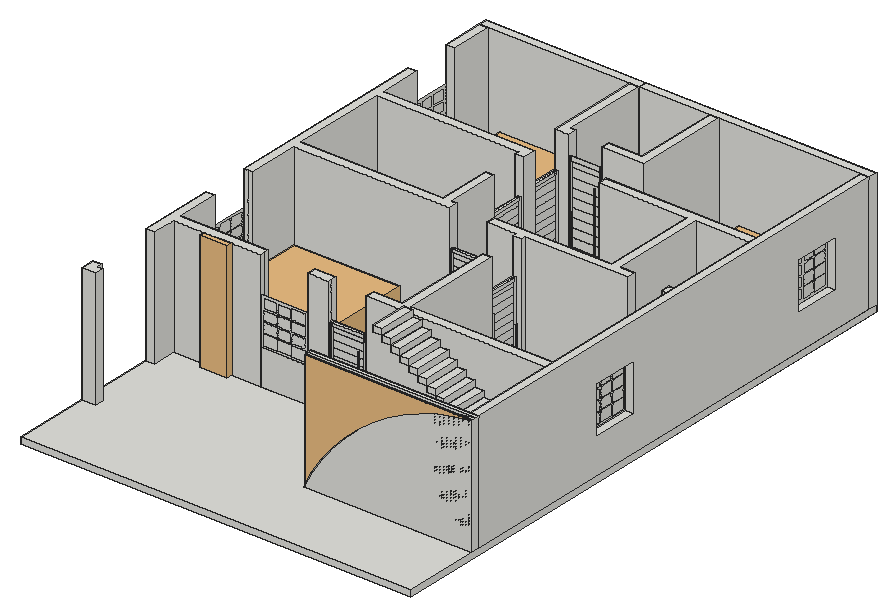
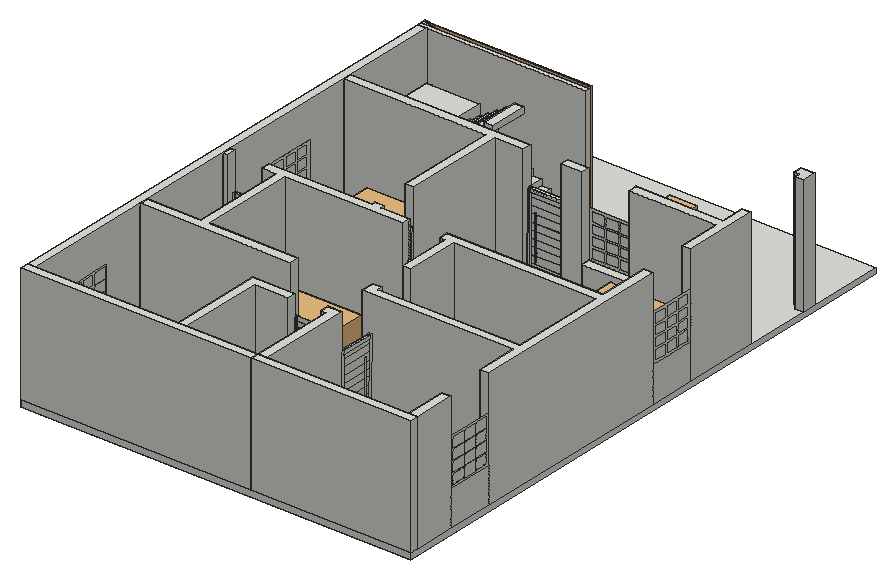
# SketchUp Ruby script. Lengths in inches.
U = 1.inch
M = Sketchup.active_model
def pt(a) = Geom::Point3d.new(a.map { |v| v * U })
def face(e, loops, mat)
  f = e.add_face(loops[0].map { |a| pt(a) })
  loops[1..].each { |l| e.add_face(l.map { |a| pt(a) }).erase! }
  f.material = f.back_material = mat if mat
  f
end
# faces: each face lists its corners as indices into pts; further lists are holes
def faces(e, pts, list, mat = nil) = list.each { |f| face(e, (f[0].is_a?(Array) ? f : [f]).map { |l| l.map { |i| pts[i] } }, mat) }
# xy, xz, yz: faces in a plane at the given z, y or x. An outline is a flat list of corners, or four numbers for a rectangle; further outlines are holes
def ring(l) = l.size == 4 ? [[l[0], l[1]], [l[2], l[1]], [l[2], l[3]], [l[0], l[3]]] : l.each_slice(2).to_a
def flat(e, list, mat, &to3) = list.each { |f| face(e, (f[0].is_a?(Array) ? f : [f]).map { |l| ring(l).map { |u, v| to3.(u, v) } }, mat) }
def xy(e, z, list, mat = nil) = flat(e, list, mat) { |x, y| [x, y, z] }
def xz(e, y, list, mat = nil) = flat(e, list, mat) { |x, z| [x, y, z] }
def yz(e, x, list, mat = nil) = flat(e, list, mat) { |y, z| [x, y, z] }
def lines(e, pts, list) = list.each { |a, b| e.add_line(pt(pts[a]), pt(pts[b])) }
# prism: a flat outline (further loops are holes) pulled along v
def prism(e, loops, v, mat = nil)
  f = face(e, loops, mat); d = Geom::Vector3d.new(v.map { |x| x * U })
  f.pushpull(f.normal.samedirection?(d) ? d.length : -d.length)
end
def box(e, o, s, mat = nil) = prism(e, [[o, [o[0] + s[0], o[1], o[2]], [o[0] + s[0], o[1] + s[1], o[2]], [o[0], o[1] + s[1], o[2]]]], [0, 0, s[2]], mat)
def at(x, y, z, deg = 0) = Geom::Transformation.translation(pt([x, y, z])) * Geom::Transformation.rotation(ORIGIN, Z_AXIS, deg.degrees)
def axes(o, x, y, z) = Geom::Transformation.new([*x, 0, *y, 0, *z, 0, *pt(o).to_a, 1])
def part(name) = M.definitions.add(name)
# library, detail: a bought-in or finely detailed component or shape, given as its bounding box
def library(name, o, s) = part(name).tap { |d| box(d.entities, o, s) }
def detail(e, o, s) = box(e.add_group.entities, o, s)
def put(e, d, t, mat = nil) = e.add_instance(d, t).tap { |i| i.material = mat if mat }
def group(e, t, mat = nil) = e.add_group.tap { |g| g.transformation = t; g.material = mat if mat }.entities
root = M.entities
c1 = part("Agrupar\#4")
xy(c1.entities,0,[[0,0,60.82,4.875]])
c2 = part("Agrupar\#7")
box(c2.entities,[0,0,0.25],[0.65,5.875,0.35])
c3 = part("Agrupar\#15")
prism(c3.entities,[[[0,0.625,0],[0.65,0.625,0],[0.65,0,0],[0,0,0]]],[0,0.02,45.16])
c4 = part("Agrupar\#14")
put(c4.entities,c2,at(0,0.65,6.88))
put(c4.entities,c3,at(0,0,0))
put(c4.entities,c2,at(0,0.65,40.25))
c5 = part("Agrupar\#6")
prism(c5.entities,[[[-0.5,0.62,-4.9375],[0.77,0.62,-4.9375],[0.77,-0.19,-4.9375],[-0.5,-0.19,-4.9375]]],[0,0.03,52.91])
c6 = part("Agrupar\#8")
put(c6.entities,c2,at(0,0.65,6.88))
put(c6.entities,c5,at(0,0,0))
put(c6.entities,c2,at(0,0.65,40.25))
c7 = part("Agrupar\#2")
prism(c7.entities,[[[0,2.67,0.04],[55.46,2.67,0.04],[55.46,0.04,0],[0,0.04,0]]],[0,-0.04,3.23])
c8 = part("Agrupar\#10")
prism(c8.entities,[[[0,3.76,0.04],[4.23,3.76,0.04],[4.23,1.14,0],[0,1.14,0]]],[0,-1.14,83.14])
c9 = part("Agrupar\#1")
prism(c9.entities,[[[0,3.76,0.04],[4.23,3.76,0.04],[4.23,1.14,0],[0,1.14,0]]],[0,-1.14,83.14])
c10 = part("Agrupar\#3")
put(c10.entities,c7,at(4.23,0,79.91))
put(c10.entities,c8,at(59.6875,0,0))
put(c10.entities,c9,at(0,0,0))
c11 = part("Agrupar\#5")
put(c11.entities,c10,axes([0,-1.34,0.11],[1,0,0],[0,3.10443,-0.05961],[0,0.0192,0.99982]))
c12 = part("Agrupar\#9")
put(c12.entities,c4,axes([49.36,10.72,17.77],[1,0,0],[0,-1,0],[0,0,1]))
put(c12.entities,c6,at(49.36,0,17.76))
put(c12.entities,c11,at(0,0.21,0.01))
c13 = part("Agrupar\#11")
box(c13.entities,[0,0,0],[60.82,4.875,7.44])
c14 = part("Agrupar\#12")
put(c14.entities,c13,at(0,0,67.34))
put(c14.entities,c13,at(0,0,44.83))
put(c14.entities,c13,at(0,0,59.9))
put(c14.entities,c13,at(0,0,74.78))
put(c14.entities,c13,at(0,0,52.37))
put(c14.entities,c13,at(0,0,7.53))
put(c14.entities,c13,at(0,0,0))
put(c14.entities,c13,at(0,0,29.95))
put(c14.entities,c13,at(0,0,15.07))
put(c14.entities,c13,at(0,0,22.51))
put(c14.entities,c13,at(0,0,37.39))
c15 = part("Agrupar\#13")
put(c15.entities,c12,at(0,0,0.0625))
put(c15.entities,c14,axes([2.375,5.17,0.15],[1,0,0],[0,0.48232,0.01095],[0,-0.02269,0.99974]))
c16 = part("PORTA PIVOTANDE ENVERNIZADA LUXURY")
p = [[59.6875,-1.28,79.91],[59.6875,-3.1,79.89],[4.23,-1.28,79.91],[4.23,-3.1,79.89]]
lines(c16.entities,p,[[0,1],[2,3]])
put(c16.entities,c1,at(0.13,-2.89,82.23))
put(c16.entities,c15,at(0,-6.8,-0.11))
c17 = library("bed",[0,0,0],[81.24,78.82,29.53])
c18 = library("SOFAS",[-9.33,-51.94,0],[132.18,168.58,37.5625])
c19 = part("Group\#19")
box(c19.entities,[0,0,0],[9,39,6])
c20 = part("Group\#20")
box(c20.entities,[0,0,0],[54,96,10])
c21 = library("Group\#143",[0,0,0],[83.17,58.86,38.65])
c22 = part("Group\#14")
xy(c22.entities,36,[[0,0,9,48]])
yz(c22.entities,0,[[0,0,48,36]])
yz(c22.entities,9,[[0,0,48,36]])
c23 = part("Group\#15")
xy(c23.entities,0,[[0,0,9,48]])
xz(c23.entities,0,[[0,0,9,36]])
xz(c23.entities,48,[[0,0,9,36]])
put(c23.entities,c22,at(0,0,0))
c24 = library("Group\#177",[0,0,0],[170.16,1.375,119.88])
c25 = part("Группа\#53")
xy(c25.entities,0,[[[-6.3,-13.1875,6.3,13.1875],[-4.25,-11.14,4.25,11.14]]])
xy(c25.entities,0.49,[[-3.9375,-10.83,3.9375,10.83]])
xy(c25.entities,0.98,[[[-6.3,-13.1875,6.3,13.1875],[-4.25,-11.14,4.25,11.14]]])
xz(c25.entities,-13.1875,[[-6.3,0,6.3,0.98]])
xz(c25.entities,-10.83,[[-3.9375,0.31,3.9375,0.49],[-3.9375,0.49,3.9375,0.67]])
xz(c25.entities,10.83,[[-3.9375,0.31,3.9375,0.49],[-3.9375,0.49,3.9375,0.67]])
xz(c25.entities,13.1875,[[-6.3,0,6.3,0.98]])
yz(c25.entities,-6.3,[[-13.1875,0,13.1875,0.98]])
yz(c25.entities,-3.9375,[[-10.83,0.31,10.83,0.49],[-10.83,0.49,10.83,0.67]])
yz(c25.entities,3.9375,[[-10.83,0.31,10.83,0.49],[-10.83,0.49,10.83,0.67]])
yz(c25.entities,6.3,[[-13.1875,0,13.1875,0.98]])
p = [[-3.9375,-10.83,0.31],[3.9375,-10.83,0.31],[-4.25,-11.14,0],[-4.25,11.14,0],[4.25,-11.14,0],[4.25,11.14,0],
  [-3.9375,10.83,0.31],[3.9375,10.83,0.31],[-3.9375,-10.83,0.67],[-3.9375,10.83,0.67],[-4.25,-11.14,0.98],[4.25,-11.14,0.98],
  [-4.25,11.14,0.98],[3.9375,-10.83,0.67],[3.9375,10.83,0.67],[4.25,11.14,0.98]]
faces(c25.entities,p,[[0,1,2],[2,3,0],[2,1,4],[5,4,1],[6,0,3],[7,5,1],[3,5,6],[7,6,5],
  [8,9,10],[10,11,8],[10,9,12],[13,8,11],[14,13,11],[14,11,15],[15,12,9],[14,15,9]])
c26 = part("Группа\#45")
xy(c26.entities,0,[[0,0,21.73,35.43]])
xy(c26.entities,29.92,[[0,0,21.73,35.43]])
xz(c26.entities,0,[[0,0,21.73,29.92]])
xz(c26.entities,35.43,[[0,0,21.73,29.92]])
yz(c26.entities,0,[[0,0,35.43,29.92]])
yz(c26.entities,21.73,[[0,0,22.44,29.92],[22.44,0,35.43,3.15],[[22.44,3.15,35.43,29.92],[22.64,3.35,35.24,29.72]]])
put(c26.entities,c25,axes([21.46,28.9375,16.54],[0,1,0],[0,0,1],[1,0,0]))
c27 = library("LIXEIRA INOX DE BANHEIRO",[-4.13,-4.13,0],[8.25,8.24,13.39])
c28 = part("Группа\#59")
xy(c28.entities,0,[[-13.1875,-4.13,13.1875,4.13]])
c29 = part("Panelled cabinet front \#2")
xy(c29.entities,0,[[[-15.55,-6.5,15.55,6.5],[-13.5,-4.45,13.5,4.45]]])
xy(c29.entities,0.98,[[[-15.55,-6.5,15.55,6.5],[-13.5,-4.45,13.5,4.45]]])
xz(c29.entities,-6.5,[[-15.55,0,15.55,0.98]])
xz(c29.entities,-4.13,[[-13.1875,0.31,13.1875,0.67]])
xz(c29.entities,4.13,[[-13.1875,0.31,13.1875,0.67]])
xz(c29.entities,6.5,[[-15.55,0,15.55,0.98]])
yz(c29.entities,-15.55,[[-6.5,0,6.5,0.98]])
yz(c29.entities,-13.1875,[[-4.13,0.31,4.13,0.67]])
yz(c29.entities,13.1875,[[-4.13,0.31,4.13,0.67]])
yz(c29.entities,15.55,[[-6.5,0,6.5,0.98]])
p = [[13.5,-4.45,0],[-13.5,-4.45,0],[13.1875,-4.13,0.31],[-13.1875,-4.13,0.31],[-13.1875,4.13,0.31],[-13.5,4.45,0],
  [13.1875,4.13,0.31],[13.5,4.45,0],[-13.5,4.45,0.98],[-13.5,-4.45,0.98],[-13.1875,-4.13,0.67],[13.5,-4.45,0.98],
  [13.1875,-4.13,0.67],[13.5,4.45,0.98],[-13.1875,4.13,0.67],[13.1875,4.13,0.67]]
faces(c29.entities,p,[[0,1,2],[3,2,1],[4,3,1],[1,5,4],[2,6,0],[0,6,7],[7,4,5],[6,4,7],
  [8,9,10],[11,10,9],[12,10,11],[11,13,12],[10,14,8],[15,12,13],[14,13,8],[14,15,13]])
put(c29.entities,c28,at(0,0,0.49))
c30 = part("Группа\#56")
xy(c30.entities,0,[[[-7.68,-13.1875,7.68,13.1875],[-5.63,-11.14,5.63,11.14]]])
xy(c30.entities,0.49,[[-5.31,-10.83,5.31,10.83]])
xy(c30.entities,0.98,[[[-7.68,-13.1875,7.68,13.1875],[-5.63,-11.14,5.63,11.14]]])
xz(c30.entities,-13.1875,[[-7.68,0,7.68,0.98]])
xz(c30.entities,-10.83,[[-5.31,0.31,5.31,0.49],[-5.31,0.49,5.31,0.67]])
xz(c30.entities,10.83,[[-5.31,0.31,5.31,0.49],[-5.31,0.49,5.31,0.67]])
xz(c30.entities,13.1875,[[-7.68,0,7.68,0.98]])
yz(c30.entities,-7.68,[[-13.1875,0,13.1875,0.98]])
yz(c30.entities,-5.31,[[-10.83,0.31,10.83,0.49],[-10.83,0.49,10.83,0.67]])
yz(c30.entities,5.31,[[-10.83,0.31,10.83,0.49],[-10.83,0.49,10.83,0.67]])
yz(c30.entities,7.68,[[-13.1875,0,13.1875,0.98]])
p = [[-5.31,-10.83,0.31],[5.31,-10.83,0.31],[-5.63,-11.14,0],[-5.63,11.14,0],[5.63,-11.14,0],[5.63,11.14,0],
  [-5.31,10.83,0.31],[5.31,10.83,0.31],[-5.31,-10.83,0.67],[-5.31,10.83,0.67],[-5.63,-11.14,0.98],[5.63,-11.14,0.98],
  [-5.63,11.14,0.98],[5.31,-10.83,0.67],[5.31,10.83,0.67],[5.63,11.14,0.98]]
faces(c30.entities,p,[[0,1,2],[2,3,0],[2,1,4],[5,4,1],[6,0,3],[7,5,1],[3,5,6],[7,6,5],
  [8,9,10],[10,11,8],[10,9,12],[13,8,11],[14,13,11],[14,11,15],[15,12,9],[14,15,9]])
c31 = part("Panelled cabinet front \#1")
xy(c31.entities,0,[[[-7.68,-13.1875,7.68,13.1875],[-5.63,-11.14,5.63,11.14]]])
xy(c31.entities,0.49,[[-5.31,-10.83,5.31,10.83]])
xy(c31.entities,0.98,[[[-7.68,-13.1875,7.68,13.1875],[-5.63,-11.14,5.63,11.14]]])
xz(c31.entities,-13.1875,[[-7.68,0,7.68,0.98]])
xz(c31.entities,-10.83,[[-5.31,0.31,5.31,0.49],[-5.31,0.49,5.31,0.67]])
xz(c31.entities,10.83,[[-5.31,0.31,5.31,0.49],[-5.31,0.49,5.31,0.67]])
xz(c31.entities,13.1875,[[-7.68,0,7.68,0.98]])
yz(c31.entities,-7.68,[[-13.1875,0,13.1875,0.98]])
yz(c31.entities,-5.31,[[-10.83,0.31,10.83,0.49],[-10.83,0.49,10.83,0.67]])
yz(c31.entities,5.31,[[-10.83,0.31,10.83,0.49],[-10.83,0.49,10.83,0.67]])
yz(c31.entities,7.68,[[-13.1875,0,13.1875,0.98]])
p = [[-5.31,-10.83,0.31],[5.31,-10.83,0.31],[-5.63,-11.14,0],[-5.63,11.14,0],[5.63,-11.14,0],[5.63,11.14,0],
  [-5.31,10.83,0.31],[5.31,10.83,0.31],[-5.63,-11.14,0.98],[5.63,-11.14,0.98],[-5.31,-10.83,0.67],[-5.31,10.83,0.67],
  [-5.63,11.14,0.98],[5.31,-10.83,0.67],[5.31,10.83,0.67],[5.63,11.14,0.98]]
faces(c31.entities,p,[[0,1,2],[2,3,0],[2,1,4],[5,4,1],[6,0,3],[7,5,1],[3,5,6],[7,6,5],
  [8,9,10],[10,11,8],[8,11,12],[13,10,9],[14,13,9],[14,9,15],[15,12,11],[14,15,11]])
c32 = part("Группа\#52")
xy(c32.entities,0,[[[-5.71,-13.1875,5.71,13.1875],[-3.66,-11.14,3.66,11.14]]])
xy(c32.entities,0.49,[[-3.35,-10.83,3.35,10.83]])
xy(c32.entities,0.98,[[[-5.71,-13.1875,5.71,13.1875],[-3.66,-11.14,3.66,11.14]]])
xz(c32.entities,-13.1875,[[-5.71,0,5.71,0.98]])
xz(c32.entities,-10.83,[[-3.35,0.31,3.35,0.49],[-3.35,0.49,3.35,0.67]])
xz(c32.entities,10.83,[[-3.35,0.31,3.35,0.49],[-3.35,0.49,3.35,0.67]])
xz(c32.entities,13.1875,[[-5.71,0,5.71,0.98]])
yz(c32.entities,-5.71,[[-13.1875,0,13.1875,0.98]])
yz(c32.entities,-3.35,[[-10.83,0.31,10.83,0.49],[-10.83,0.49,10.83,0.67]])
yz(c32.entities,3.35,[[-10.83,0.31,10.83,0.49],[-10.83,0.49,10.83,0.67]])
yz(c32.entities,5.71,[[-13.1875,0,13.1875,0.98]])
p = [[3.66,-11.14,0],[-3.66,-11.14,0],[-3.35,-10.83,0.31],[-3.66,11.14,0],[3.35,-10.83,0.31],[3.66,11.14,0],
  [-3.35,10.83,0.31],[3.35,10.83,0.31],[-3.66,11.14,0.98],[-3.66,-11.14,0.98],[-3.35,10.83,0.67],[-3.35,-10.83,0.67],
  [3.35,-10.83,0.67],[3.66,-11.14,0.98],[3.35,10.83,0.67],[3.66,11.14,0.98]]
faces(c32.entities,p,[[0,1,2],[3,2,1],[4,0,2],[5,0,4],[6,2,3],[7,5,4],[3,5,6],[7,6,5],
  [8,9,10],[11,10,9],[12,11,9],[12,9,13],[14,12,13],[13,15,14],[10,14,8],[8,14,15]])
c33 = part("Группа\#54")
xy(c33.entities,0,[[[-6.4,-13.1875,6.4,13.1875],[-4.35,-11.14,4.35,11.14]]])
xy(c33.entities,0.49,[[-4.04,-10.83,4.04,10.83]])
xy(c33.entities,0.98,[[[-6.4,-13.1875,6.4,13.1875],[-4.35,-11.14,4.35,11.14]]])
xz(c33.entities,-13.1875,[[-6.4,0,6.4,0.98]])
xz(c33.entities,-10.83,[[-4.04,0.31,4.04,0.49],[-4.04,0.49,4.04,0.67]])
xz(c33.entities,10.83,[[-4.04,0.31,4.04,0.49],[-4.04,0.49,4.04,0.67]])
xz(c33.entities,13.1875,[[-6.4,0,6.4,0.98]])
yz(c33.entities,-6.4,[[-13.1875,0,13.1875,0.98]])
yz(c33.entities,-4.04,[[-10.83,0.31,10.83,0.49],[-10.83,0.49,10.83,0.67]])
yz(c33.entities,4.04,[[-10.83,0.31,10.83,0.49],[-10.83,0.49,10.83,0.67]])
yz(c33.entities,6.4,[[-13.1875,0,13.1875,0.98]])
p = [[4.35,-11.14,0],[-4.35,-11.14,0],[-4.04,-10.83,0.31],[-4.04,10.83,0.31],[-4.35,11.14,0],[4.04,-10.83,0.31],
  [4.35,11.14,0],[4.04,10.83,0.31],[-4.35,11.14,0.98],[-4.35,-11.14,0.98],[-4.04,-10.83,0.67],[4.35,-11.14,0.98],
  [4.04,-10.83,0.67],[4.35,11.14,0.98],[-4.04,10.83,0.67],[4.04,10.83,0.67]]
faces(c33.entities,p,[[0,1,2],[3,2,1],[1,4,3],[5,0,2],[6,0,7],[5,7,0],[6,3,4],[7,3,6],
  [8,9,10],[11,10,9],[12,10,11],[13,12,11],[10,14,8],[15,12,13],[13,8,15],[14,15,8]])
c34 = library("Inodoro ROCA Meridian-N compact",[-14.68,0,0],[14.68,23.62,31.16])
c35 = library("Grupo\#25",[0.45,21.05,9.1],[4.32,4.21,6.93])
c36 = library("00230906_3D_ducha_hig.dwg\#1",[121.96,-107.5,-116.36],[35.26,104.03,274.49])
c37 = library("Gruppe\#2",[0,-1.9,0],[31.7,22.18,26.07])
c38 = part("Группа\#84")
prism(c38.entities,[[[-19.46,0,0],[-144,0,0],[-144,47.24,0],[-120.375,47.24,0],[-120.375,23.62,0],[-19.46,23.62,0]],[[-81.02,2.55,0],[-81.02,20.78,0],[-106.12,20.78,0],[-106.12,2.55,0]]],[0,0,1.57])
c39 = library("Group\#136",[0,0,0],[7.4375,14.82,1.97])
c40 = library("Group\#138",[0,0,0],[10.4375,12.4,1.97])
c41 = library("Group\#135",[0,0,0],[5.12,5.12,1.0625])
c42 = library("Group\#137",[0,0,0],[7.4375,14.82,1.97])
c43 = part("window_2")
xz(c43.entities,0,[[[-16,0,16,41],[-14,30.25,-5.25,39],[5.25,30.25,14,39],[5.25,2,14,10.75],[-14,2,-5.25,10.75],[-4.25,30.25,4.25,39],[-4.25,2,4.25,10.75],[5.25,21,14,29.25],[5.25,11.75,14,20],[-14,21,-5.25,29.25],[-14,11.75,-5.25,20],[-4.25,21,4.25,29.25],[-4.25,11.75,4.25,20]],[-14,2,-5.25,10.75],[-4.25,2,4.25,10.75],[5.25,2,14,10.75],[-14,11.75,-5.25,20],
  [-4.25,11.75,4.25,20],[5.25,11.75,14,20],[-14,21,-5.25,29.25],[-4.25,21,4.25,29.25],[5.25,21,14,29.25],
  [-14,30.25,-5.25,39],[-4.25,30.25,4.25,39],[5.25,30.25,14,39]])
c44 = library("Gruppe\#1",[0,0,0],[10.625,1.33,3.5625])
c45 = part("Component\#35")
detail(c45.entities,[0,0,0],[0.1,0.79,0.125])
c46 = library("Component\#38",[0,0,0],[0.16,0.16,0.04])
prism(root,[[[52.638,387.274,41.253],[52.658,387.274,41.25],[52.679,387.274,41.253],[52.698,387.274,41.261],[52.714,387.274,41.273],[52.726,387.274,41.289],[52.734,387.274,41.308],[52.737,387.274,41.329],[52.734,387.274,41.349],[52.726,387.274,41.368],[52.714,387.274,41.384],[52.698,387.274,41.397],[52.679,387.274,41.405],[52.658,387.274,41.407],[52.638,387.274,41.405],[52.619,387.274,41.397],[52.602,387.274,41.384],[52.59,387.274,41.368],[52.582,387.274,41.349],[52.579,387.274,41.329],[52.582,387.274,41.308],[52.59,387.274,41.289],[52.602,387.274,41.273],[52.619,387.274,41.261]]],[0,-0.002,0])
prism(root,[[[56.178,387.274,41.263],[56.199,387.274,41.26],[56.219,387.274,41.263],[56.238,387.274,41.27],[56.254,387.274,41.283],[56.267,387.274,41.299],[56.275,387.274,41.318],[56.278,387.274,41.339],[56.275,387.274,41.359],[56.267,387.274,41.378],[56.254,387.274,41.394],[56.238,387.274,41.407],[56.219,387.274,41.415],[56.199,387.274,41.417],[56.178,387.274,41.415],[56.159,387.274,41.407],[56.143,387.274,41.394],[56.131,387.274,41.378],[56.123,387.274,41.359],[56.12,387.274,41.339],[56.123,387.274,41.318],[56.131,387.274,41.299],[56.143,387.274,41.283],[56.159,387.274,41.27]]],[0,-0.002,0])
prism(root,[[[59.719,387.274,41.272],[59.739,387.274,41.27],[59.76,387.274,41.272],[59.779,387.274,41.28],[59.795,387.274,41.293],[59.808,387.274,41.309],[59.816,387.274,41.328],[59.818,387.274,41.348],[59.816,387.274,41.369],[59.808,387.274,41.388],[59.795,387.274,41.404],[59.779,387.274,41.417],[59.76,387.274,41.424],[59.739,387.274,41.427],[59.719,387.274,41.424],[59.7,387.274,41.417],[59.684,387.274,41.404],[59.671,387.274,41.388],[59.663,387.274,41.369],[59.661,387.274,41.348],[59.663,387.274,41.328],[59.671,387.274,41.309],[59.684,387.274,41.293],[59.7,387.274,41.28]]],[0,-0.002,0])
xy(root,0,[[257.25,120,428.25,129]])
xy(root,26.378,[[109.514,386.793,109.675,386.814,109.825,386.876,109.954,386.975,110.052,387.104,110.115,387.254,110.136,387.415,110.115,387.576,110.052,387.726,109.954,387.855,109.825,387.954,109.675,388.016,109.514,388.037,109.353,388.016,109.203,387.954,109.074,387.855,108.975,387.726,108.913,387.576,108.892,387.415,108.913,387.254,108.975,387.104,109.074,386.975,109.203,386.876,109.353,386.814]])
xy(root,26.772,[[[109.514,386.628,109.718,386.654,109.908,386.733,110.071,386.858,110.196,387.021,110.274,387.211,110.301,387.415,110.274,387.619,110.196,387.809,110.071,387.972,109.908,388.097,109.718,388.176,109.514,388.202,109.31,388.176,109.12,388.097,108.957,387.972,108.832,387.809,108.753,387.619,108.726,387.415,108.753,387.211,108.832,387.021,108.957,386.858,109.12,386.733,109.31,386.654],[109.514,386.793,109.353,386.814,109.203,386.876,109.074,386.975,108.975,387.104,108.913,387.254,108.892,387.415,108.913,387.576,108.975,387.726,109.074,387.855,109.203,387.954,109.353,388.016,109.514,388.037,109.675,388.016,109.825,387.954,109.954,387.855,110.052,387.726,110.115,387.576,110.136,387.415,110.115,387.254,110.052,387.104,109.954,386.975,109.825,386.876,109.675,386.814]]])
xy(root,120,[[257.25,124.5625,428.25,129]])
xz(root,120,[[257.25,0,428.25,0,428.25,120,410.262,117.372,392.561,113.229,375.275,107.599,358.529,100.525,342.443,92.056,327.133,82.255,312.709,71.19,299.274,58.942,286.927,45.6,275.755,31.259,265.839,16.022]])
xz(root,124.5625,[[257.25,0,265.839,16.022,275.755,31.259,286.927,45.6,299.274,58.942,312.709,71.19,327.133,82.255,342.443,92.056,358.529,100.525,375.275,107.599,392.561,113.229,410.262,117.372,428.25,120,257.25,120]])
xz(root,129,[[257.25,0,428.25,120]])
xz(root,422.433,[[41.25,0,62.982,3.15],[41.25,3.15,62.982,29.921]])
xz(root,534,[[32.25,0,41.25,36]])
xz(root,582,[[32.25,0,41.25,36]])
yz(root,62.982,[[[422.433,3.15,434.244,29.921],[422.63,3.346,434.047,29.724]]])
yz(root,143.548,[[405.828,32.839,405.823,32.841,405.97,33.413,405.975,33.411],[405.823,32.841,404.574,33.161,404.721,33.733,405.97,33.413]])
yz(root,143.862,[[405.826,32.84,405.973,33.412,405.97,33.413,405.823,32.841],[405.823,32.841,405.97,33.413,404.717,33.734,404.57,33.162]])
yz(root,257.25,[[124.5625,0,129,120]])
yz(root,428.25,[[120,0,129,120]])
p = [[257.25,120,0],[265.839,120,16.022],[265.839,124.5625,16.022],[257.25,124.5625,0],[275.755,120,31.259],[275.755,124.5625,31.259],
  [109.203,386.876,26.772],[109.353,386.814,26.772],[109.353,386.814,26.378],[109.203,386.876,26.378],[109.514,386.793,26.772],[109.514,386.793,26.378],
  [109.675,386.814,26.772],[109.675,386.814,26.378],[109.825,386.876,26.772],[109.825,386.876,26.378],[109.074,386.975,26.772],[109.074,386.975,26.378],
  [109.954,386.975,26.772],[109.954,386.975,26.378],[108.975,387.104,26.772],[108.975,387.104,26.378],[110.052,387.104,26.772],[110.052,387.104,26.378],
  [108.913,387.254,26.772],[108.913,387.254,26.378],[110.115,387.254,26.772],[110.115,387.254,26.378],[108.892,387.415,26.772],[108.892,387.415,26.378],
  [110.136,387.415,26.772],[110.136,387.415,26.378],[108.913,387.576,26.772],[108.913,387.576,26.378],[110.115,387.576,26.772],[110.115,387.576,26.378],
  [108.975,387.726,26.772],[108.975,387.726,26.378],[110.052,387.726,26.772],[110.052,387.726,26.378],[109.074,387.855,26.772],[109.074,387.855,26.378],
  [109.954,387.855,26.772],[109.954,387.855,26.378],[109.203,387.954,26.772],[109.203,387.954,26.378],[109.825,387.954,26.772],[109.825,387.954,26.378],
  [109.353,388.016,26.772],[109.353,388.016,26.378],[109.514,388.037,26.772],[109.514,388.037,26.378],[109.675,388.016,26.772],[109.675,388.016,26.378],
  [286.927,120,45.6],[286.927,124.5625,45.6],[143.114,404.798,32.697],[143.054,404.957,32.657],[143.037,405.125,32.613],[143.066,405.292,32.571],
  [143.139,405.446,32.531],[143.25,405.577,32.498],[143.393,405.675,32.472],[143.557,405.734,32.457],[143.73,405.75,32.453],[143.903,405.721,32.46],
  [144.062,405.651,32.478],[144.196,405.543,32.506],[144.297,405.405,32.542],[144.358,405.246,32.582],[144.375,405.078,32.626],[144.346,404.911,32.668],
  [144.273,404.757,32.708],[144.162,404.627,32.741],[144.019,404.529,32.767],[143.855,404.47,32.782],[143.681,404.454,32.786],[143.509,404.482,32.779],
  [143.35,404.553,32.76],[143.216,404.66,32.733],[144.297,405.503,32.923],[144.358,405.344,32.964],[143.066,405.39,32.952],[143.139,405.544,32.912],
  [143.25,405.674,32.879],[144.196,405.641,32.887],[144.062,405.749,32.86],[143.393,405.773,32.854],[143.548,405.828,32.839],[143.557,405.832,32.839],
  [143.573,405.834,32.838],[143.573,405.98,33.41],[143.705,405.992,33.407],[143.705,405.845,32.835],[143.73,405.847,32.834],[143.758,405.843,32.836],
  [143.758,405.99,33.408],[143.862,405.973,33.412],[143.862,405.826,32.84],[143.903,405.819,32.842],[144.375,405.176,33.007],[144.346,405.009,33.05],
  [143.054,405.055,33.038],[143.037,405.223,32.995],[144.162,404.725,33.123],[144.019,404.627,33.148],[143.35,404.65,33.142],[143.216,404.758,33.114],
  [144.273,404.855,33.089],[143.114,404.896,33.079],[143.509,404.58,33.16],[143.681,404.552,33.167],[143.652,404.557,33.166],[143.652,404.703,33.738],
  [143.548,404.721,33.733],[143.548,404.574,33.161],[143.855,404.568,33.163],[143.837,404.565,33.164],[143.837,404.712,33.736],[143.705,404.701,33.739],
  [143.705,404.554,33.167],[143.862,404.57,33.162],[143.548,405.823,32.841],[143.862,405.823,32.841],[143.548,405.975,33.411],[143.732,405.844,32.835],
  [143.732,405.991,33.407],[143.678,404.555,33.166],[143.678,404.702,33.738],[143.862,404.717,33.734],[143.548,405.97,33.413],[143.862,405.97,33.413],
  [299.274,120,58.942],[299.274,124.5625,58.942],[312.709,120,71.19],[312.709,124.5625,71.19],[327.133,120,82.255],[327.133,124.5625,82.255],
  [342.443,120,92.056],[342.443,124.5625,92.056],[358.529,120,100.525],[358.529,124.5625,100.525],[375.275,120,107.599],[375.275,124.5625,107.599],
  [392.561,120,113.229],[392.561,124.5625,113.229],[410.262,120,117.372],[410.262,124.5625,117.372],[428.25,120,120],[428.25,124.5625,120],
  [143.573,404.568,33.163],[143.626,404.559,33.165],[143.599,404.563,33.164],[143.784,404.558,33.166],[143.758,404.555,33.166],[143.81,404.561,33.165],
  [143.731,404.554,33.167],[143.548,404.565,33.164],[138.024,405.837,32.837],[137.998,405.841,32.836],[137.971,405.843,32.836],[137.945,405.844,32.835],
  [137.918,405.844,32.835],[135.738,404.51,32.771],[135.905,404.465,32.783],[135.594,405.613,32.488],[135.471,405.495,32.518],[136.068,405.841,32.836],
  [136.042,405.843,32.836],[135.912,405.739,32.456],[135.745,405.696,32.467],[136.016,405.844,32.835],[135.384,405.351,32.556],[135.989,405.844,32.835],
  [136.396,404.59,32.751],[136.519,404.708,32.721],[136.606,404.853,32.683],[143.862,404.565,33.164],[135.589,404.594,32.75],[135.381,404.859,32.682],
  [135.467,404.713,32.719],[136.609,405.344,32.557],[136.523,405.49,32.52],[136.652,405.015,32.642],[136.653,405.182,32.599],[136.252,405.694,32.467],
  [136.085,405.738,32.456],[136.402,405.609,32.489],[136.078,404.464,32.783],[136.246,404.507,32.772],[135.337,405.021,32.64],[135.338,405.189,32.597],
  [153.59,405.961,32.48],[153.588,405.882,32.48],[136.092,405.838,32.837],[56.267,387.276,41.299],[56.267,387.274,41.299],[56.254,387.276,41.394],
  [56.254,387.274,41.394],[56.238,387.276,41.27],[56.238,387.274,41.27],[56.159,387.276,41.407],[56.159,387.274,41.407],[56.275,387.276,41.359],
  [56.275,387.274,41.359],[56.123,387.276,41.318],[56.123,387.274,41.318],[56.278,387.276,41.339],[56.278,387.274,41.339],[56.254,387.276,41.283],
  [56.254,387.274,41.283],[56.131,387.276,41.378],[56.131,387.274,41.378],[56.267,387.276,41.378],[56.267,387.274,41.378],[56.123,387.276,41.359],
  [56.123,387.274,41.359],[56.219,387.276,41.263],[56.219,387.274,41.263],[56.143,387.276,41.394],[56.143,387.274,41.394],[56.238,387.276,41.407],
  [56.238,387.274,41.407],[56.219,387.276,41.415],[56.219,387.274,41.415],[56.199,387.276,41.26],[56.199,387.274,41.26],[56.178,387.276,41.415],
  [56.178,387.274,41.415],[56.199,387.276,41.417],[56.199,387.274,41.417],[56.178,387.276,41.263],[56.178,387.274,41.263],[56.143,387.276,41.283],
  [56.143,387.274,41.283],[56.12,387.276,41.339],[56.12,387.274,41.339],[56.159,387.276,41.27],[56.159,387.274,41.27],[56.275,387.276,41.318],
  [56.275,387.274,41.318],[56.131,387.276,41.299],[56.131,387.274,41.299],[143.6,405.838,32.837],[143.679,405.845,32.835],[143.652,405.844,32.835],
  [143.626,405.841,32.836],[143.837,405.832,32.839],[143.811,405.836,32.837],[143.784,405.84,32.836],[41.25,624,0],[41.25,624,120],
  [32.25,624,0],[32.25,624,120],[59.795,387.276,41.404],[59.795,387.274,41.404],[59.779,387.276,41.417],[59.779,387.274,41.417],
  [59.7,387.276,41.28],[59.7,387.274,41.28],[59.816,387.276,41.369],[59.816,387.274,41.369],[59.739,387.276,41.27],[59.739,387.274,41.27],
  [59.671,387.276,41.309],[59.671,387.274,41.309],[59.739,387.276,41.427],[59.739,387.274,41.427],[59.795,387.276,41.293],[59.795,387.274,41.293],
  [59.779,387.276,41.28],[59.779,387.274,41.28],[59.76,387.276,41.272],[59.76,387.274,41.272],[59.7,387.276,41.417],[59.7,387.274,41.417],
  [59.684,387.276,41.404],[59.684,387.274,41.404],[59.663,387.276,41.369],[59.663,387.274,41.369],[59.816,387.276,41.328],[59.816,387.274,41.328],
  [59.808,387.276,41.388],[59.808,387.274,41.388],[59.76,387.276,41.424],[59.76,387.274,41.424],[59.671,387.276,41.388],[59.671,387.274,41.388],
  [59.719,387.276,41.272],[59.719,387.274,41.272],[59.719,387.276,41.424],[59.719,387.274,41.424],[59.818,387.276,41.348],[59.818,387.274,41.348],
  [59.808,387.276,41.309],[59.808,387.274,41.309],[59.684,387.276,41.293],[59.684,387.274,41.293],[59.663,387.276,41.328],[59.663,387.274,41.328],
  [59.661,387.276,41.348],[59.661,387.274,41.348],[52.734,387.276,41.349],[52.734,387.274,41.349],[52.619,387.276,41.397],[52.619,387.274,41.397],
  [52.714,387.276,41.384],[52.714,387.274,41.384],[52.698,387.276,41.397],[52.698,387.274,41.397],[52.579,387.276,41.329],[52.579,387.274,41.329],
  [52.638,387.276,41.253],[52.638,387.274,41.253],[52.658,387.276,41.407],[52.658,387.274,41.407],[52.679,387.276,41.405],[52.679,387.274,41.405],
  [52.582,387.276,41.308],[52.582,387.274,41.308],[52.59,387.276,41.368],[52.59,387.274,41.368],[52.658,387.276,41.25],[52.658,387.274,41.25],
  [52.734,387.276,41.308],[52.734,387.274,41.308],[52.619,387.276,41.261],[52.619,387.274,41.261],[52.602,387.276,41.384],[52.602,387.274,41.384],
  [52.737,387.276,41.329],[52.737,387.274,41.329],[52.59,387.276,41.289],[52.59,387.274,41.289],[52.698,387.276,41.261],[52.698,387.274,41.261],
  [52.714,387.276,41.273],[52.714,387.274,41.273],[52.726,387.276,41.368],[52.726,387.274,41.368],[52.726,387.276,41.289],[52.726,387.274,41.289],
  [52.679,387.276,41.253],[52.679,387.274,41.253],[52.582,387.276,41.349],[52.582,387.274,41.349],[52.638,387.276,41.405],[52.638,387.274,41.405],
  [52.602,387.276,41.273],[52.602,387.274,41.273]]
faces(root,p,[[0,1,2,3],[1,4,5,2],[6,7,8,9],[7,10,11,8],[10,12,13,11],[12,14,15,13],[16,6,9,17],[14,18,19,15],
  [20,16,17,21],[18,22,23,19],[24,20,21,25],[22,26,27,23],[28,24,25,29],[26,30,31,27],[32,28,29,33],[30,34,35,31],
  [36,32,33,37],[34,38,39,35],[40,36,37,41],[38,42,43,39],[44,40,41,45],[42,46,47,43],[48,44,45,49],[50,48,49,51],
  [52,50,51,53],[46,52,53,47],[4,54,55,5],[56,57,58,59,60,61,62,63,64,65,66,67,68,69,70,71,72,73,74,75,76,77,78,79],[69,68,80,81],[60,59,82,83],[61,60,83,84],[68,67,85,80],
  [67,66,86,85],[62,61,84,87],[63,62,87,88,89],[64,63,89,90,91,92,93,94],[65,64,94,95,96,97,98,99],[66,65,99,86],[71,70,100,101],[58,57,102,103],
  [59,58,103,82],[70,69,81,100],[74,73,104,105],[79,78,106,107],[73,72,108,104],[56,79,107,109],[57,56,109,102],[72,71,101,108],
  [78,77,110,106],[77,76,111,112,113,114,115,110],[76,75,116,117,118,119,120,111],[75,74,105,121,116],[110,115,122,88,87,84,83,82,103,102,109,107,106],[99,98,123,121,105,104,108,101,100,81,80,85,86],[90,88,124,91],[125,93,92,126],
  [95,125,126,96],[127,120,119,128],[112,127,128,113],[117,121,129,118],[97,96,126,92,91,124,130,114,113,128,119,118,129,131],[54,132,133,55],[132,134,135,133],[134,136,137,135],
  [136,138,139,137],[138,140,141,139],[140,142,143,141],[142,144,145,143],[144,146,147,145],[146,148,149,147]])
lines(root,p,[[150,115],[112,151],[151,152],[152,150],[153,154],[117,155],[155,153],[154,156],[156,120],[157,115],[158,159],[159,160],
  [160,161],[161,162],[163,164],[165,166],[167,168],[169,170],[168,171],[166,172],[171,173],[174,175],[175,176],[121,177],
  [178,163],[179,180],[181,182],[183,184],[185,186],[187,185],[182,187],[180,178],[170,165],[184,181],[176,183],[186,169],
  [188,189],[190,179],[191,190],[172,191],[164,188],[189,174],[192,193],[194,167],[195,196],[197,198],[199,200],[201,202],
  [203,204],[205,206],[207,208],[209,210],[211,212],[213,214],[215,216],[217,218],[219,220],[221,222],[223,224],[225,226],
  [227,228],[229,230],[231,232],[233,234],[235,236],[237,238],[239,240],[241,242],[243,90],[93,244],[244,245],[245,246],
  [246,243],[98,247],[247,248],[248,249],[249,95],[250,251],[252,253],[254,255],[256,257],[258,259],[260,261],[262,263],
  [264,265],[266,267],[268,269],[270,271],[272,273],[274,275],[276,277],[278,279],[280,281],[282,283],[284,285],[286,287],
  [288,289],[290,291],[292,293],[294,295],[296,297],[298,299],[300,301],[302,303],[304,305],[306,307],[308,309],[310,311],
  [312,313],[314,315],[316,317],[318,319],[320,321],[322,323],[324,325],[326,327],[328,329],[330,331],[332,333],[334,335],
  [336,337],[338,339],[340,341],[342,343],[344,345],[346,347],[348,349]])
detail(root,[62.98,387,0],[123.94,23.56,29.92])
detail(root,[72.5,219,0],[27.4375,6,120])
detail(root,[168.23,409.44,14.6],[5.89,1.12,1.51])
detail(root,[97.58,409.44,27.85],[5.89,1.12,1.51])
detail(root,[81.83,409.44,27.85],[5.89,1.12,1.51])
detail(root,[112.84,409.44,27.86],[5.89,1.12,1.52])
detail(root,[67.18,409.44,27.97],[5.89,1.12,1.51])
detail(root,[168.23,409.44,27.98],[5.89,1.12,1.52])
detail(root,[63.69,425.39,27.98],[1.12,5.89,1.52])
detail(root,[124.77,389.74,31.5],[30.2,18.11,1.77])
detail(root,[137.26,404.46,32.45],[1.33,1.53,1.29])
detail(root,[135.33,404.46,32.45],[1.33,1.53,1.29])
detail(root,[141.11,404.46,32.45],[1.33,1.53,1.29])
detail(root,[139.18,404.46,32.45],[1.33,1.53,1.29])
detail(root,[50.89,386.02,39.56],[10.62,1.29,3.56])
detail(root,[51.63,387.22,40.31],[2.05,0.13,2.04])
detail(root,[55.17,387.22,40.31],[2.05,0.13,2.05])
detail(root,[58.71,387.22,40.32],[2.05,0.13,2.05])
g1 = group(root,at(32.25,120,-6))
box(g1,[0,-78.125,0],[396,591.125,6])
put(root,c16,axes([186.83,529.3125,0.11],[0,-0.5895,0],[0.36,0,0],[0,0,1]))
put(root,c17,at(395.25,234,0,90))
g2 = group(root,at(185.25,529.3125,0))
xy(g2,0,[[0,0,0,94.6875,9,94.6875,9,9,14,9,14,0],[46.9375,0,46.9375,8.8125,81,8.8125,81,94.6875,90,94.6875,90,0]])
xy(g2,120,[[0,0,14,0,14,9,9,9,9,94.6875,0,94.6875],[46.9375,0,90,0,90,94.6875,81,94.6875,81,8.8125,46.9375,8.8125]])
xz(g2,0,[[0,0,14,120],[46.9375,0,90,120]])
xz(g2,8.8125,[[46.9375,0,81,120]])
xz(g2,9,[[9,0,14,120]])
xz(g2,94.6875,[[0,0,9,120],[81,0,90,120]])
yz(g2,0,[[0,0,94.6875,120]])
yz(g2,9,[[9,0,94.6875,120]])
yz(g2,14,[[0,0,9,120]])
yz(g2,46.9375,[[0,0,8.8125,120]])
yz(g2,81,[[8.8125,0,94.6875,120]])
yz(g2,90,[[0,0,94.6875,120]])
g3 = group(root,at(32.25,120,0))
prism(g3,[[[14,0,0],[0,0,0],[0,14,0],[9,14,0],[9,9,0],[14,9,0]]],[0,0,120])
put(root,c16,axes([199.25,530.13,0.18],[0.51535,0,0],[0,0.10352,0],[0,0,1.21]))
put(root,c18,axes([140.76,333.63,0],[-0.81,0,0],[0,-0.85419,0],[0,0,0.81]))
g4 = group(root,at(32.25,582,0))
box(g4,[0,0,0],[9,42,120])
g5 = group(root,at(237.26,373.93,0))
box(g5,[176.99,4.07,0],[5,9,120])
xy(g5,0,[[28.99,0,28.99,4.07,0,4.07,0,13.07,142.49,13.07,142.49,4.07,37.99,4.07,37.99,0],[118.99,13.07,118.99,109.07,28.99,109.07,28.99,118.07,181.99,118.07,181.99,109.07,127.99,109.07,127.99,13.07]])
xy(g5,120,[[28.99,0,37.99,0,37.99,4.07,142.49,4.07,142.49,13.07,127.99,13.07,127.99,109.07,181.99,109.07,181.99,118.07,28.99,118.07,28.99,109.07,118.99,109.07,118.99,13.07,0,13.07,0,4.07,28.99,4.07]])
xz(g5,0,[[28.99,0,37.99,120]])
xz(g5,4.07,[[0,0,28.99,120],[37.99,0,142.49,120]])
xz(g5,13.07,[[0,0,118.99,120],[127.99,0,142.49,120]])
xz(g5,109.07,[[28.99,0,118.99,120],[127.99,0,181.99,120]])
xz(g5,118.07,[[28.99,0,181.99,120]])
yz(g5,0,[[4.07,0,5.1,120],[5.1,0,13.07,120]])
yz(g5,28.99,[[0,0,4.07,120],[109.07,0,118.07,120]])
yz(g5,37.99,[[0,0,4.07,120]])
yz(g5,118.99,[[13.07,0,109.07,120]])
yz(g5,127.99,[[13.07,0,109.07,120]])
yz(g5,142.49,[[4.07,0,13.07,120]])
yz(g5,181.99,[[109.07,0,118.07,120]])
g6 = group(root,at(275.25,129,0))
put(g6,c19,at(0,57,118))
put(g6,c19,at(63,57,76))
put(g6,c19,at(81,57,64))
put(g6,c19,at(0,0,0))
put(g6,c19,at(18,0,12))
put(g6,c19,at(9,0,6))
put(g6,c19,at(36,0,24))
put(g6,c19,at(27,0,18))
put(g6,c19,at(81,0,54))
put(g6,c19,at(72,57,70))
put(g6,c19,at(45,57,88))
put(g6,c19,at(72,0,48))
put(g6,c19,at(54,0,36))
put(g6,c19,at(27,57,100))
put(g6,c19,at(18,57,106))
put(g6,c19,at(9,57,112))
put(g6,c19,at(63,0,42))
put(g6,c20,at(90,0,60))
put(g6,c19,at(45,0,30))
put(g6,c19,at(54,57,82))
put(g6,c19,at(36,57,94))
put(root,c21,at(260,410.61,0))
g7 = group(root,at(236.93,225,0))
xy(g7,0,[[0,0,0,9,29.32,9,29.32,110.82,38.32,110.82,38.32,9,182.32,9,182.32,0]])
xy(g7,120,[[0,0,182.32,0,182.32,9,38.32,9,38.32,110.82,29.32,110.82,29.32,9,0,9]])
xz(g7,0,[[0,0,182.32,120]])
xz(g7,9,[[0,0,29.32,120],[38.32,0,182.32,120]])
xz(g7,110.82,[[29.32,0,38.32,120]])
yz(g7,0,[[0,0,9,120]])
yz(g7,29.32,[[9,0,110.82,120]])
yz(g7,38.32,[[9,0,110.82,120]])
yz(g7,182.32,[[0,0,9,120]])
g8 = group(root,at(266.25,624,0))
box(g8,[-72,0,0],[234,9,120])
g9 = group(root,at(32.25,201,0))
prism(g9,[[[9,76.5,0],[9,33,0],[97.5,33,0],[97.5,28.5,0],[97.5,24,0],[9,24,0],[9,0,0],[0,0,0],[0,76.5,0]]],[0,0,120])
put(root,c23,at(32.25,277.5,0))
put(root,c23,at(32.25,534,0))
g10 = group(root,at(419.25,129,0))
prism(g10,[[[0,495,0],[0,0,0],[0,0,120],[0,495,120]],[[0,405,84],[0,405,36],[0,453,36],[0,453,84]],[[0,196.5,36],[0,196.5,84],[0,148.5,84],[0,148.5,36]]],[9,0,0])
put(root,c23,at(177.75,225,0,90))
g11 = group(root,at(32.25,624,0))
box(g11,[0,0,0],[162,9,120])
g12 = group(root,at(177.75,225,0))
prism(g12,[[[21.5,0,0],[0,0,0],[0,9,0],[21.5,9,0],[21.5,2.72,0]]],[0,0,120])
g13 = group(root,at(32.25,325.5,0))
xy(g13,0,[[0,0,9,208.5],[9,52.5,9,61.5,153,61.5,153,115.1875,162,115.1875,162,61.5,167,61.5,167,52.5],[153,152.5,153,157.5,9,157.5,9,166.5,162,166.5,162,152.5]])
xy(g13,120,[[0,0,9,0,9,52.5,167,52.5,167,61.5,162,61.5,162,115.1875,153,115.1875,153,61.5,9,61.5,9,157.5,153,157.5,153,152.5,162,152.5,162,166.5,9,166.5,9,208.5,0,208.5]])
xz(g13,0,[[0,0,4.5,120],[4.5,0,9,120]])
xz(g13,52.5,[[9,0,167,120]])
xz(g13,61.5,[[9,0,153,120],[162,0,167,120]])
xz(g13,115.1875,[[153,0,162,120]])
xz(g13,152.5,[[153,0,162,120]])
xz(g13,157.5,[[9,0,153,120]])
xz(g13,166.5,[[9,0,162,120]])
xz(g13,208.5,[[0,0,9,120]])
yz(g13,0,[[0,0,208.5,120]])
yz(g13,9,[[0,0,52.5,120],[61.5,0,157.5,120],[166.5,0,208.5,120]])
yz(g13,153,[[61.5,0,115.1875,120],[152.5,0,157.5,120]])
yz(g13,162,[[61.5,0,115.1875,120],[152.5,0,166.5,120]])
yz(g13,167,[[52.5,0,61.5,120]])
put(root,c16,axes([199.25,227.85,0.15],[0.5895,0,0],[0,0.36,0],[0,0,1]))
put(root,c16,axes([379.75,380.94,0.15],[0.5398,0,0],[0,0.37131,0],[0,0,1]))
put(root,c16,axes([199.25,380.28,0.15],[0.5895,0,0],[0,0.36,0],[0,0,1]))
put(root,c16,axes([190.88,478.36,0.15],[0,-0.5895,0],[0.36,0,0],[0,0,1]))
put(root,c16,axes([273.28,529.68,0.15],[0,-0.5895,0],[0.36,0,0],[0,0,1]))
put(root,c16,axes([269.1,373.5,0.15],[0,-0.5895,0],[0.36,0,0],[0,0,1]))
put(root,c17,at(296.25,624,0,-90))
put(root,c24,at(258.09,120,0))
put(root,c17,at(53.35,624,0,-90))
put(root,c26,at(41.25,387,0))
put(root,c27,axes([255.69,557.07,1.14],[-0.00004,-0.93528,-0.0057],[0.93528,0,-0.00588],[0.00447,-0.00433,0.7108]))
put(root,c29,axes([171.17,408.46,9.84],[-1,0,0],[0,0,1],[0,1,0]))
put(root,c30,axes([116.05,408.46,16.54],[-1,0,0],[0,0,1],[0,1,0]))
put(root,c31,axes([100.31,408.46,16.54],[-1,0,0],[0,0,1],[0,1,0]))
put(root,c31,axes([84.56,408.46,16.54],[-1,0,0],[0,0,1],[0,1,0]))
put(root,c32,axes([62.71,428.34,16.54],[0,1,0],[0,0,1],[1,0,0]))
put(root,c33,axes([70.09,408.46,16.54],[-1,0,0],[0,0,1],[0,1,0]))
put(root,c28,axes([139.68,408.95,9.84],[-1,0,0],[0,0,1],[0,1,0]))
put(root,c34,axes([266.05,575.4375,7.33],[0.00004,0.99998,0.00609],[-0.99998,0,0.00628],[0.00628,-0.00609,0.99996]))
put(root,c35,axes([266.6,602.01,1.16],[-0.99998,0,0.00628],[-0.00004,-0.99998,-0.00609],[0.00628,-0.00609,0.99996]))
put(root,c36,axes([277.76,553.51,25.14],[-0.09516,0,0.0006],[0,-0.05567,-0.00034],[0.0006,-0.00058,0.09516]))
put(root,c29,axes([171.17,408.46,23.23],[-1,0,0],[0,0,1],[0,1,0]))
put(root,c28,axes([139.68,408.95,23.23],[-1,0,0],[0,0,1],[0,1,0]))
put(root,c37,at(72.53,388.57,22.6))
put(root,c38,at(185.25,387,29.92))
put(root,c39,axes([153.3125,391.39,34.17],[-1,0,0],[0,1,0],[0,0,-1]))
put(root,c40,axes([134.65,403.8,34.17],[1,0,0],[0,-1,0],[0,0,-1]))
put(root,c41,at(142.43,399.58,32.2,180))
put(root,c42,axes([126.42,406.21,34.17],[1,0,0],[0,-1,0],[0,0,-1]))
put(root,c43,axes([153.75,225,36],[1.5,0,0],[0,1.17,0],[0,0,1.17]))
put(root,c43,axes([32.25,301.5,36],[0,-1.5,0],[1.17,0,0],[0,0,1.17]))
put(root,c43,axes([419.25,558,36],[0,-1.5,0],[1.17,0,0],[0,0,1.17]))
put(root,c43,axes([32.25,558,36],[0,-1.5,0],[1.17,0,0],[0,0,1.17]))
put(root,c43,axes([419.25,301.5,36],[0,-1.5,0],[1.17,0,0],[0,0,1.17]))
put(root,c44,at(181.34,387.35,39.56,180))
put(root,c45,axes([52.71,387.34,40.61],[-1,0,0],[0,-0.11,0],[0,0,-1]))
put(root,c45,axes([56.25,387.34,40.62],[-1,0,0],[0,-0.11,0],[0,0,-1]))
put(root,c45,axes([59.79,387.34,40.63],[-1,0,0],[0,-0.11,0],[0,0,-1]))
put(root,c46,axes([52.74,387.27,41.25],[-1,0,0],[0,0,1],[0,0.11,0]))
put(root,c46,axes([56.28,387.27,41.26],[-1,0,0],[0,0,1],[0,0.11,0]))
put(root,c46,axes([59.82,387.27,41.27],[-1,0,0],[0,0,1],[0,0.11,0]))
put(root,c45,axes([52.71,387.34,42.05],[-1,0,0],[0,-0.11,0],[0,0,1]))
put(root,c45,axes([56.25,387.34,42.06],[-1,0,0],[0,-0.11,0],[0,0,1]))
put(root,c45,axes([59.79,387.34,42.07],[-1,0,0],[0,-0.11,0],[0,0,1]))
